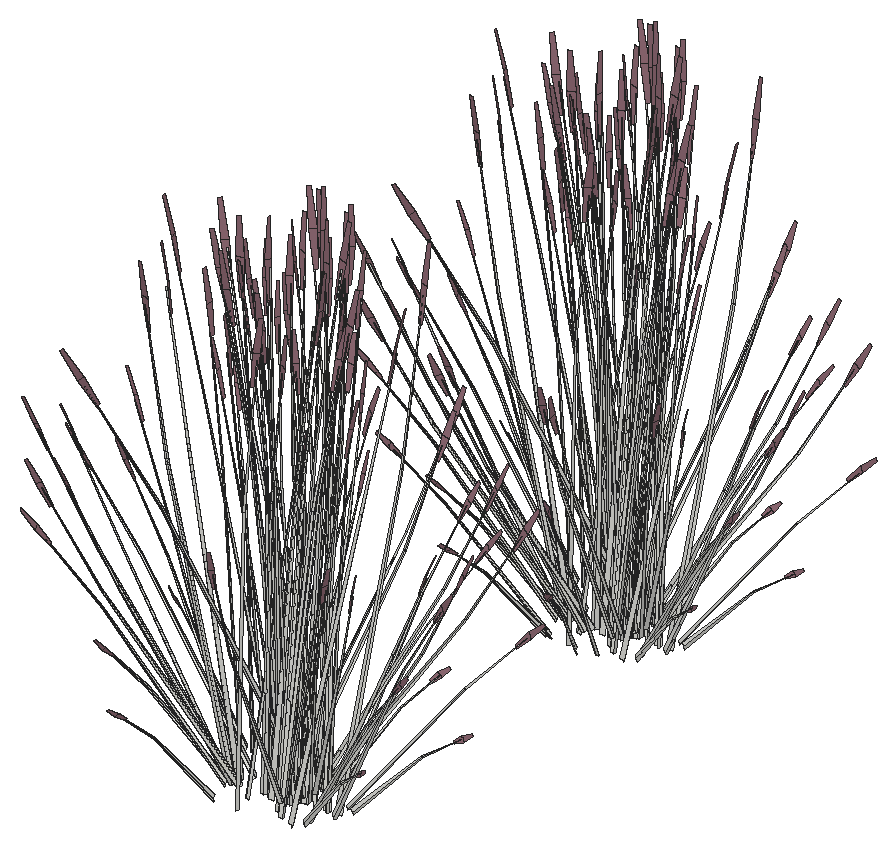
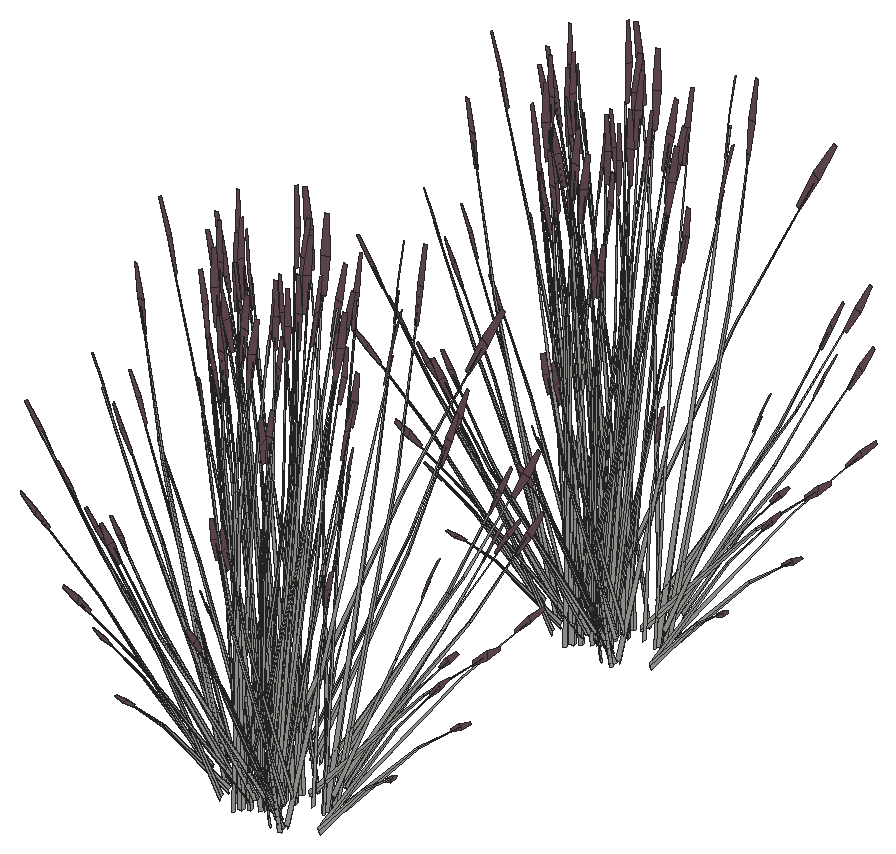
# SketchUp Ruby script. Lengths in inches.
U = 1.inch
M = Sketchup.active_model
def pt(a) = Geom::Point3d.new(a.map { |v| v * U })
def face(e, loops, mat)
  f = e.add_face(loops[0].map { |a| pt(a) })
  loops[1..].each { |l| e.add_face(l.map { |a| pt(a) }).erase! }
  f.material = f.back_material = mat if mat
  f
end
# faces: each face lists its corners as indices into pts; further lists are holes
def faces(e, pts, list, mat = nil) = list.each { |f| face(e, (f[0].is_a?(Array) ? f : [f]).map { |l| l.map { |i| pts[i] } }, mat) }
# xy, xz, yz: faces in a plane at the given z, y or x. An outline is a flat list of corners, or four numbers for a rectangle; further outlines are holes
def ring(l) = l.size == 4 ? [[l[0], l[1]], [l[2], l[1]], [l[2], l[3]], [l[0], l[3]]] : l.each_slice(2).to_a
def flat(e, list, mat, &to3) = list.each { |f| face(e, (f[0].is_a?(Array) ? f : [f]).map { |l| ring(l).map { |u, v| to3.(u, v) } }, mat) }
def xy(e, z, list, mat = nil) = flat(e, list, mat) { |x, y| [x, y, z] }
def xz(e, y, list, mat = nil) = flat(e, list, mat) { |x, z| [x, y, z] }
def yz(e, x, list, mat = nil) = flat(e, list, mat) { |y, z| [x, y, z] }
def lines(e, pts, list) = list.each { |a, b| e.add_line(pt(pts[a]), pt(pts[b])) }
# prism: a flat outline (further loops are holes) pulled along v
def prism(e, loops, v, mat = nil)
  f = face(e, loops, mat); d = Geom::Vector3d.new(v.map { |x| x * U })
  f.pushpull(f.normal.samedirection?(d) ? d.length : -d.length)
end
def box(e, o, s, mat = nil) = prism(e, [[o, [o[0] + s[0], o[1], o[2]], [o[0] + s[0], o[1] + s[1], o[2]], [o[0], o[1] + s[1], o[2]]]], [0, 0, s[2]], mat)
def at(x, y, z, deg = 0) = Geom::Transformation.translation(pt([x, y, z])) * Geom::Transformation.rotation(ORIGIN, Z_AXIS, deg.degrees)
def axes(o, x, y, z) = Geom::Transformation.new([*x, 0, *y, 0, *z, 0, *pt(o).to_a, 1])
def part(name) = M.definitions.add(name)
# library, detail: a bought-in or finely detailed component or shape, given as its bounding box
def library(name, o, s) = part(name).tap { |d| box(d.entities, o, s) }
def detail(e, o, s) = box(e.add_group.entities, o, s)
def put(e, d, t, mat = nil) = e.add_instance(d, t).tap { |i| i.material = mat if mat }
def group(e, t, mat = nil) = e.add_group.tap { |g| g.transformation = t; g.material = mat if mat }.entities
root = M.entities
M.materials.add("LightPink_Translucent").color = [144, 107, 117]
c1 = part("blade")
p = [[2.15,0.21,22],[0,0.17,0],[0.09,0.45,0],[2.18,0.31,22],[2.29,0.31,22],[0.38,0.45,0],
  [2.48,0.24,33],[2.49,0.24,33],[2.48,0.22,33]]
faces(c1.entities,p,[[0,1,2,3],[4,5,2,3],[6,3,4,7],[8,0,3,6]])
c2 = part("seeds")
p = [[0.3,-0.1,1.38],[-0.01,-0.03,1.59],[-0.01,-0.03,0.03],[0.14,-0.07,-0.07],[0.29,-0.03,3],[0.15,0.01,3.11]]
faces(c2.entities,p,[[0,1,2,3],[1,0,4,5]],"LightPink_Translucent")
c3 = part("blade with seeds")
put(c3.entities,c1,at(0,0,0))
put(c3.entities,c2,axes([2.4,0.25,30.99],[1.5799,-0.05474,1.17369],[-0.12525,1.92788,0.29478],[-0.07173,-0.02425,1.56792]))
put(root,c3,axes([55.18,640.24,46.68],[-0.87728,-0.69587,-0.51099],[0.92674,-0.60943,-0.3958],[0.13348,-0.35356,0.97773]))
put(root,c3,axes([48.84,638.0625,44.77],[0.63926,0.36046,1.1486],[-0.93099,0.21668,0.84392],[-0.1992,-0.27702,0.25299]))
put(root,c3,axes([50.39,639.97,46.98],[-1.04497,-0.50058,-0.71045],[0.74264,-0.8772,0.08574],[-0.3786,-0.29889,1.00501]))
put(root,c3,axes([49.9,640,46.68],[-1.20928,0.24619,-0.51099],[-0.21154,-0.93233,-0.3958],[-0.32481,-0.26718,0.97773]))
put(root,c3,axes([57.04,642.22,46.98],[0.64013,-0.81717,-0.71045],[1.12174,0.58074,0.08574],[0.38221,-0.29607,1.00501]))
put(root,c3,axes([50.12,639.84,44.375],[-0.7662,-1.03778,0],[1.28187,-0.57875,-0.51607],[0.29196,-0.13181,1.63711]))
put(root,c3,axes([57.01,641.84,46.68],[-0.31482,-0.94565,-0.51099],[1.19224,-0.16542,-0.3958],[0.34166,-0.254,0.97773]))
put(root,c3,axes([52.89,645.64,45.33],[1.05902,0.41762,1.51261],[-1.03748,0.89969,0.59816],[-0.46471,-0.53324,1.26806]))
put(root,c3,axes([57.97,641.47,44.59],[-0.4378,-0.03068,1.43002],[-0.44851,-0.8229,-0.30754],[0.53783,-0.23279,0.61141]))
put(root,c3,axes([58.47,639.96,44.77],[-0.40819,0.5272,1.1486],[-0.35086,-0.70831,0.84392],[0.33713,-0.17749,0.25299]))
put(root,c3,axes([47.01,643.53,44.375],[-1.53239,0,0],[0,-1.1575,-0.51607],[0,-0.26363,1.63711]))
put(root,c3,axes([47.27,641.47,44.59],[0.23927,0.28834,1.43002],[-0.55135,0.78376,-0.30754],[-0.56612,-0.18733,0.61141]))
put(root,c3,axes([48.26,641.21,46.98],[-1.22504,-0.02494,-0.71045],[0.08228,-1.05005,0.08574],[-0.51899,-0.11081,1.00501]))
put(root,c3,axes([48.19,643.23,44.33],[-1.1399,0.87071,0.30756],[-1.1406,-0.86155,-0.36492],[-0.03981,-0.24727,1.64885]))
put(root,c3,axes([51.82,643.63,44.43],[1.3808,0.50196,0.24065],[-0.66454,1.04299,0.50002],[0,-0.24043,1.60543]))
put(root,c3,axes([47.85,641.42,46.68],[-0.88986,0.68603,-0.51099],[-0.77932,-0.72471,-0.3958],[-0.45212,-0.10438,0.97773]))
put(root,c3,axes([45.84,642.33,44.77],[0.78239,-0.07411,1.1486],[-0.49629,0.65296,0.84392],[-0.38663,-0.09795,0.25299]))
put(root,c3,axes([51.375,642.94,44.72],[-1.33077,0.06393,0.44739],[-0.12035,-1.06125,-0.21531],[0.23824,-0.10756,1.43643]))
put(root,c3,axes([47.9375,643.71,44.48],[0,1.03566,0.49651],[-1.37109,0,0],[0,-0.23588,1.57504]))
put(root,c3,axes([57.5625,643.94,46.68],[0.332,-0.94205,-0.51099],[1.13828,0.3229,-0.3958],[0.45829,-0.08638,0.97773]))
put(root,c3,axes([55.76,640.1,44.375],[0.7662,-1.03778,0],[1.28187,0.57875,-0.51607],[0.29196,0.13181,1.63711]))
put(root,c3,axes([51.33,643.32,44.36],[0.53281,1.15808,0.45755],[-1.52239,0.4027,0.17955],[0.01861,-0.2128,1.58856]))
put(root,c3,axes([58.78,644.21,43.98],[-0.7893,0.12429,1.41583],[-0.12563,-0.9893,0.08104],[0.55282,-0.14974,0.80566]))
put(root,c3,axes([51.06,644.23,44.72],[-0.59459,0.93321,0.44739],[-1.23546,-0.44912,-0.21531],[0,-0.21512,1.43643]))
put(root,c3,axes([53.24,643.42,44.21],[0,-1.19833,0],[1.53239,0,0],[0,0,1.79456]))
put(root,c3,axes([55.1,640.65,44.48],[-1.14694,-0.51783,0.49651],[0.68554,-0.92854,0],[0.26122,0.11794,1.57504]))
put(root,c3,axes([57.34,644.28,46.98],[1.07686,-0.45739,-0.71045],[0.60013,0.94154,0.08574],[0.52031,-0.10696,1.00501]))
put(root,c3,axes([52.52,642.66,44.36],[-1.01611,0.93987,0.45755],[-1.20717,-0.82966,0.17955],[0.24496,-0.0938,1.58856]))
put(root,c3,axes([53.625,644.34,44.3],[-1.1399,-0.8914,-0.06131],[1.1406,-0.89194,0],[-0.03981,-0.03113,1.75571]))
put(root,c3,axes([50.75,641.11,44.47],[-0.35402,1.02926,0.17642],[-1.29548,-0.29127,0.35086],[0.22379,-0.00501,1.60407]))
put(root,c3,axes([53.46,642.26,44.62],[0.23642,-0.92427,0.1448],[1.15506,0.16044,-0.41347],[0.21021,0.09491,1.26744]))
put(root,c3,axes([51.46,644.45,44.36],[1.54892,0.2182,0.45755],[-0.31522,1.23236,0.17955],[-0.22636,-0.119,1.58856]))
put(root,c3,axes([52.96,642.5,44.72],[-0.73619,-0.86927,0.44739],[1.11511,-0.61213,-0.21531],[0.23824,0.10756,1.43643]))
put(root,c3,axes([50.63,646.42,44.47],[1.31687,-0.27488,0.17642],[0.32517,1.02297,0.35086],[-0.11745,-0.14905,1.60407]))
put(root,c3,axes([54.28,643.68,44.21],[1.37109,0,0],[0,1.07219,0],[0,0,1.78407]))
put(root,c3,axes([54.67,641.17,44.47],[-1.31687,0.27488,0.17642],[-0.32517,-1.02297,0.35086],[0.11745,0.14905,1.60407]))
put(root,c3,axes([53.84,643.14,44.38],[-1.54892,-0.2182,0.49198],[0.31522,-1.23236,0.19306],[0.22636,0.119,1.70813]))
put(root,c3,axes([52.61,646.18,44.2],[-0.39985,-0.89288,0],[1.1418,-0.31268,0],[0,0,1.54371]))
put(root,c3,axes([51.84,645.33,44.62],[-0.23642,0.92427,0.1448],[-1.15506,-0.16044,-0.41347],[-0.21021,-0.09491,1.26744]))
put(root,c3,axes([54.55,646.48,44.47],[0.35402,-1.02926,0.17642],[1.29548,0.29127,0.35086],[-0.22379,0.00501,1.60407]))
put(root,c3,axes([54.25,644.14,44.21],[0.85545,0.66896,0],[-0.85545,0.66896,0],[0,0,1.69266]))
put(root,c3,axes([49.39,642.89,45.34],[0.34834,-0.14982,1.77064],[0.12012,1.04605,0.13857],[-0.75452,0.1388,0.63284]))
put(root,c3,axes([56.57,643.85,44.47],[-0.96285,-0.75439,0.17642],[0.97031,-0.7317,0.35086],[-0.10634,0.15406,1.60407]))
put(root,c3,axes([60.42,644.54,44.77],[-0.75718,0.17097,1.1486],[0.35641,-0.70661,0.84392],[0.40168,0.04835,0.25299]))
put(root,c3,axes([52.32,646.58,44.2],[-1.23546,-0.46496,0],[0.59459,-0.96613,0],[0,0,1.62707]))
put(root,c3,axes([50.2,646.94,44.48],[1.14694,0.51783,0.49651],[-0.68554,0.92854,0],[-0.26122,-0.11794,1.57504]))
put(root,c3,axes([54.24,643.36,44.72],[0.59459,-0.93321,0.44739],[1.23546,0.44912,-0.21531],[0,0.21512,1.43643]))
put(root,c3,axes([54.01,643.89,44.29],[0,1.19774,-0.05637],[-1.53239,0,0],[0,0.03764,1.79368]))
put(root,c3,axes([46.99,643.46,46.68],[-0.332,0.94205,-0.51099],[-1.13828,-0.3229,-0.3958],[-0.45829,0.08638,0.97773]))
put(root,c3,axes([49.54,647.49,44.375],[-0.7662,1.03778,0],[-1.28187,-0.57875,-0.51607],[-0.29196,-0.13181,1.63711]))
put(root,c3,axes([57.36,643.88,44.48],[0,-1.03566,0.49651],[1.37109,0,0],[0,0.23588,1.57504]))
put(root,c3,axes([53.93,644.66,44.72],[1.33077,-0.06393,0.44739],[0.12035,1.06125,-0.21531],[-0.23824,0.10756,1.43643]))
put(root,c3,axes([54.76,643.57,44.62],[1.1418,-0.30203,0.1448],[0.39985,0.86246,-0.41347],[0,0.18981,1.26744]))
put(root,c3,axes([59,645.68,44.59],[-0.29514,-0.25472,1.43002],[0.38401,-0.84262,-0.30754],[0.59714,0.11414,0.61141]))
put(root,c3,axes([53.72,646.6,44.2],[1.23546,0.46496,0],[-0.59459,0.96613,0],[0,0,1.74954]))
put(root,c3,axes([54.22,647.63,44.19],[-0.75665,-1.04141,-0.05142],[1.28187,-0.57875,0.51607],[-0.31588,0.09915,1.6363]))
put(root,c3,axes([53.95,645.11,44.62],[0.90538,0.62224,0.1448],[-0.75521,0.70202,-0.41347],[-0.21021,0.09491,1.26744]))
put(root,c3,axes([56.29,646.1875,46.98],[1.22504,0.02494,-0.71045],[-0.08228,1.05005,0.08574],[0.51899,0.11081,1.00501]))
put(root,c3,axes([54.91,647.03,44.48],[1.14694,-0.51783,0.49651],[0.68554,0.92854,0],[-0.26122,0.11794,1.57504]))
put(root,c3,axes([53.28,646.21,44.29],[0.53281,1.18979,-0.06012],[-1.52239,0.41691,0],[0.01861,0.04155,1.72173]))
put(root,c3,axes([45.62,645.67,44.59],[0.42589,0.08502,1.43002],[0.2745,0.86839,-0.30754],[-0.57851,0.16255,0.61141]))
put(root,c3,axes([58.29,644.06,44.375],[1.53239,0,0],[0,1.1575,-0.51607],[0,0.26363,1.63711]))
put(root,c3,axes([57.68,644.65,44.2],[-1.53164,-0.00828,-0.04976],[0,-1.1575,0.49943],[-0.04813,0.2635,1.58352]))
put(root,c3,axes([44.73,647.49,44.77],[0.51072,-0.46938,1.1486],[0.20153,0.74307,0.84392],[-0.36908,0.13305,0.25299]))
put(root,c3,axes([54.25,647.1,44.33],[1.53422,0.33662,0.30756],[-0.38383,1.20322,-0.36492],[-0.25393,0.15059,1.64885]))
put(root,c3,axes([56.21,646.99,44.77],[-0.69001,-0.29779,1.1486],[0.89096,-0.30257,0.84392],[0.24031,0.2563,0.25299]))
put(root,c3,axes([47.54,645.56,46.68],[0.31482,0.94565,-0.51099],[-1.19224,0.16542,-0.3958],[-0.34166,0.254,0.97773]))
put(root,c3,axes([55.18,647.75,44.375],[0.7662,1.03778,0],[-1.28187,0.57875,-0.51607],[-0.29196,0.13181,1.63711]))
put(root,c3,axes([54.53,643.64,44.84],[-0.03348,-0.97511,1.41272],[1.51511,0.25277,0.59816],[-0.35835,0.53357,1.3335]))
put(root,c3,axes([54.65,647.4,46.68],[1.20928,-0.24619,-0.51099],[0.21154,0.93233,-0.3958],[0.32481,0.26718,0.97773]))
put(root,c3,axes([56.32,648.35,44.67],[-0.78586,-0.03248,1.0506],[0.51898,-0.68985,0.58006],[0.31045,0.24509,0.8241]))
put(root,c3,axes([53.75,646.67,44.59],[0.02163,-0.34331,1.43002],[1.03345,-0.38348,-0.30754],[0.31903,0.4109,0.61141]))
put(root,c3,axes([49.07,649.53,44.77],[-0.03171,-0.6158,1.1486],[0.7925,0.43922,0.84392],[-0.15586,0.29352,0.25299]))
put(root,c3,axes([49.36,647.16,47],[0.87728,0.69587,-0.5672],[-0.92674,0.60943,-0.43934],[-0.13348,0.35356,1.08528]))
put(root,c3,axes([48.41,648.2,44.82],[1.11329,-0.1834,0.06507],[0.25594,0.73887,-0.86304],[-0.07058,0.37403,0.7736]))
put(root,c3,axes([51.96,647.83,46.68],[1.20468,0.25962,-0.51099],[-0.41292,0.89013,-0.3958],[0.11046,0.35838,0.97773]))
put(root,c3,axes([49.09,646.84,47.34],[-0.03189,0.95798,-0.7886],[-1.34277,-0.06434,0.09517],[-0.14171,0.40585,1.11556]))
put(root,c3,axes([51.53,647.66,46.98],[0.5849,0.8421,-0.71045],[-1.20401,0.4693,0.08574],[0.13677,0.40688,1.00501]))
put(root,c3,axes([48.14,648.99,44.59],[0.38672,-0.16338,1.43002],[0.95481,0.49262,-0.30754],[-0.28419,0.42626,0.61141]))
put(root,c3,axes([48.64,648.19,45.36],[0.02693,-0.53464,1.54345],[1.21102,0.2824,0.21329],[-0.10493,0.5698,0.72882]))
put(root,c3,axes([59.15,683.33,44.59],[-0.34835,0.20963,1.43002],[-1.04325,-0.36691,-0.30754],[0.19338,-0.4563,0.61141]))
put(root,c3,axes([57.5625,684.0625,46.98],[-0.5849,-0.8421,-0.71045],[1.20401,-0.4693,0.08574],[-0.13677,-0.40688,1.00501]))
put(root,c3,axes([53.76,682.9375,44.59],[-0.07421,0.33879,1.43002],[-1.08488,0.28361,-0.30754],[-0.25359,-0.4379,0.61141]))
put(root,c3,axes([60,684.89,46.98],[0.03189,-0.95798,-0.71045],[1.34277,0.06434,0.08574],[0.14171,-0.40585,1.00501]))
put(root,c3,axes([57.12,683.89,46.68],[-1.20468,-0.25962,-0.51099],[0.41292,-0.89013,-0.3958],[-0.11046,-0.35838,0.97773]))
put(root,c3,axes([57.87,681.66,44.77],[0.15721,0.60392,1.1486],[-0.87211,-0.33448,0.84392],[0.09385,-0.30923,0.25299]))
put(root,c3,axes([59.72,684.57,46.68],[-0.87728,-0.69587,-0.51099],[0.92674,-0.60943,-0.3958],[0.13348,-0.35356,0.97773]))
put(root,c3,axes([53.38,682.39,44.77],[0.63926,0.36046,1.1486],[-0.93099,0.21668,0.84392],[-0.1992,-0.27702,0.25299]))
put(root,c3,axes([54.93,684.3,46.98],[-1.04497,-0.50058,-0.71045],[0.74264,-0.8772,0.08574],[-0.3786,-0.29889,1.00501]))
put(root,c3,axes([54.4375,684.33,46.68],[-1.20928,0.24619,-0.51099],[-0.21154,-0.93233,-0.3958],[-0.32481,-0.26718,0.97773]))
put(root,c3,axes([61.58,686.55,46.98],[0.64013,-0.81717,-0.71045],[1.12174,0.58074,0.08574],[0.38221,-0.29607,1.00501]))
put(root,c3,axes([54.66,684.17,44.375],[-0.7662,-1.03778,0],[1.28187,-0.57875,-0.51607],[0.29196,-0.13181,1.63711]))
put(root,c3,axes([61.55,686.17,46.68],[-0.31482,-0.94565,-0.51099],[1.19224,-0.16542,-0.3958],[0.34166,-0.254,0.97773]))
put(root,c3,axes([57.43,689.96,45.33],[1.05902,0.41762,1.51261],[-1.03748,0.89969,0.59816],[-0.46471,-0.53324,1.26806]))
put(root,c3,axes([62.51,685.8,44.59],[-0.4378,-0.03068,1.43002],[-0.44851,-0.8229,-0.30754],[0.53783,-0.23279,0.61141]))
put(root,c3,axes([63.01,684.29,44.77],[-0.40819,0.5272,1.1486],[-0.35086,-0.70831,0.84392],[0.33713,-0.17749,0.25299]))
put(root,c3,axes([51.55,687.86,44.375],[-1.53239,0,0],[0,-1.1575,-0.51607],[0,-0.26363,1.63711]))
put(root,c3,axes([51.81,685.79,44.59],[0.23927,0.28834,1.43002],[-0.55135,0.78376,-0.30754],[-0.56612,-0.18733,0.61141]))
put(root,c3,axes([52.8,685.54,46.98],[-1.22504,-0.02494,-0.71045],[0.08228,-1.05005,0.08574],[-0.51899,-0.11081,1.00501]))
put(root,c3,axes([52.73,687.56,44.33],[-1.1399,0.87071,0.30756],[-1.1406,-0.86155,-0.36492],[-0.03981,-0.24727,1.64885]))
put(root,c3,axes([56.36,687.96,44.43],[1.3808,0.50196,0.24065],[-0.66454,1.04299,0.50002],[0,-0.24043,1.60543]))
put(root,c3,axes([52.39,685.75,46.68],[-0.88986,0.68603,-0.51099],[-0.77932,-0.72471,-0.3958],[-0.45212,-0.10438,0.97773]))
put(root,c3,axes([50.38,686.66,44.77],[0.78239,-0.07411,1.1486],[-0.49629,0.65296,0.84392],[-0.38663,-0.09795,0.25299]))
put(root,c3,axes([55.91,687.26,44.72],[-1.33077,0.06393,0.44739],[-0.12035,-1.06125,-0.21531],[0.23824,-0.10756,1.43643]))
put(root,c3,axes([52.48,688.04,44.48],[0,1.03566,0.49651],[-1.37109,0,0],[0,-0.23588,1.57504]))
put(root,c3,axes([62.1,688.27,46.68],[0.332,-0.94205,-0.51099],[1.13828,0.3229,-0.3958],[0.45829,-0.08638,0.97773]))
put(root,c3,axes([60.3,684.43,44.375],[0.7662,-1.03778,0],[1.28187,0.57875,-0.51607],[0.29196,0.13181,1.63711]))
put(root,c3,axes([55.87,687.65,44.36],[0.53281,1.15808,0.45755],[-1.52239,0.4027,0.17955],[0.01861,-0.2128,1.58856]))
put(root,c3,axes([63.32,688.53,43.98],[-0.7893,0.12429,1.41583],[-0.12563,-0.9893,0.08104],[0.55282,-0.14974,0.80566]))
put(root,c3,axes([55.6,688.56,44.72],[-0.59459,0.93321,0.44739],[-1.23546,-0.44912,-0.21531],[0,-0.21512,1.43643]))
put(root,c3,axes([57.78,687.74,44.21],[0,-1.19833,0],[1.53239,0,0],[0,0,1.79456]))
put(root,c3,axes([59.64,684.98,44.48],[-1.14694,-0.51783,0.49651],[0.68554,-0.92854,0],[0.26122,0.11794,1.57504]))
put(root,c3,axes([61.88,688.61,46.98],[1.07686,-0.45739,-0.71045],[0.60013,0.94154,0.08574],[0.52031,-0.10696,1.00501]))
put(root,c3,axes([57.06,686.99,44.36],[-1.01611,0.93987,0.45755],[-1.20717,-0.82966,0.17955],[0.24496,-0.0938,1.58856]))
put(root,c3,axes([58.17,688.67,44.3],[-1.1399,-0.8914,-0.06131],[1.1406,-0.89194,0],[-0.03981,-0.03113,1.75571]))
put(root,c3,axes([55.29,685.44,44.47],[-0.35402,1.02926,0.17642],[-1.29548,-0.29127,0.35086],[0.22379,-0.00501,1.60407]))
put(root,c3,axes([58,686.59,44.62],[0.23642,-0.92427,0.1448],[1.15506,0.16044,-0.41347],[0.21021,0.09491,1.26744]))
put(root,c3,axes([56,688.78,44.36],[1.54892,0.2182,0.45755],[-0.31522,1.23236,0.17955],[-0.22636,-0.119,1.58856]))
put(root,c3,axes([57.5,686.83,44.72],[-0.73619,-0.86927,0.44739],[1.11511,-0.61213,-0.21531],[0.23824,0.10756,1.43643]))
put(root,c3,axes([55.17,690.75,44.47],[1.31687,-0.27488,0.17642],[0.32517,1.02297,0.35086],[-0.11745,-0.14905,1.60407]))
put(root,c3,axes([58.82,688.01,44.21],[1.37109,0,0],[0,1.07219,0],[0,0,1.78407]))
put(root,c3,axes([59.21,685.5,44.47],[-1.31687,0.27488,0.17642],[-0.32517,-1.02297,0.35086],[0.11745,0.14905,1.60407]))
put(root,c3,axes([58.38,687.47,44.38],[-1.54892,-0.2182,0.49198],[0.31522,-1.23236,0.19306],[0.22636,0.119,1.70813]))
put(root,c3,axes([57.15,690.51,44.2],[-0.39985,-0.89288,0],[1.1418,-0.31268,0],[0,0,1.54371]))
put(root,c3,axes([56.38,689.66,44.62],[-0.23642,0.92427,0.1448],[-1.15506,-0.16044,-0.41347],[-0.21021,-0.09491,1.26744]))
put(root,c3,axes([59.09,690.81,44.47],[0.35402,-1.02926,0.17642],[1.29548,0.29127,0.35086],[-0.22379,0.00501,1.60407]))
put(root,c3,axes([58.79,688.47,44.21],[0.85545,0.66896,0],[-0.85545,0.66896,0],[0,0,1.69266]))
put(root,c3,axes([53.93,687.22,45.34],[0.34834,-0.14982,1.77064],[0.12012,1.04605,0.13857],[-0.75452,0.1388,0.63284]))
put(root,c3,axes([61.11,688.18,44.47],[-0.96285,-0.75439,0.17642],[0.97031,-0.7317,0.35086],[-0.10634,0.15406,1.60407]))
put(root,c3,axes([64.96,688.87,44.77],[-0.75718,0.17097,1.1486],[0.35641,-0.70661,0.84392],[0.40168,0.04835,0.25299]))
put(root,c3,axes([56.86,690.91,44.2],[-1.23546,-0.46496,0],[0.59459,-0.96613,0],[0,0,1.62707]))
put(root,c3,axes([54.74,691.27,44.48],[1.14694,0.51783,0.49651],[-0.68554,0.92854,0],[-0.26122,-0.11794,1.57504]))
put(root,c3,axes([58.78,687.6875,44.72],[0.59459,-0.93321,0.44739],[1.23546,0.44912,-0.21531],[0,0.21512,1.43643]))
put(root,c3,axes([58.55,688.22,44.29],[0,1.19774,-0.05637],[-1.53239,0,0],[0,0.03764,1.79368]))
put(root,c3,axes([51.53,687.79,46.68],[-0.332,0.94205,-0.51099],[-1.13828,-0.3229,-0.3958],[-0.45829,0.08638,0.97773]))
put(root,c3,axes([54.08,691.81,44.375],[-0.7662,1.03778,0],[-1.28187,-0.57875,-0.51607],[-0.29196,-0.13181,1.63711]))
put(root,c3,axes([61.9,688.21,44.48],[0,-1.03566,0.49651],[1.37109,0,0],[0,0.23588,1.57504]))
put(root,c3,axes([58.47,688.98,44.72],[1.33077,-0.06393,0.44739],[0.12035,1.06125,-0.21531],[-0.23824,0.10756,1.43643]))
put(root,c3,axes([59.3,687.9,44.62],[1.1418,-0.30203,0.1448],[0.39985,0.86246,-0.41347],[0,0.18981,1.26744]))
put(root,c3,axes([63.54,690,44.59],[-0.29514,-0.25472,1.43002],[0.38401,-0.84262,-0.30754],[0.59714,0.11414,0.61141]))
put(root,c3,axes([58.26,690.93,44.2],[1.23546,0.46496,0],[-0.59459,0.96613,0],[0,0,1.74954]))
put(root,c3,axes([58.76,691.96,44.19],[-0.75665,-1.04141,-0.05142],[1.28187,-0.57875,0.51607],[-0.31588,0.09915,1.6363]))
put(root,c3,axes([58.49,689.44,44.62],[0.90538,0.62224,0.1448],[-0.75521,0.70202,-0.41347],[-0.21021,0.09491,1.26744]))
put(root,c3,axes([60.83,690.52,46.98],[1.22504,0.02494,-0.71045],[-0.08228,1.05005,0.08574],[0.51899,0.11081,1.00501]))
put(root,c3,axes([59.45,691.36,44.48],[1.14694,-0.51783,0.49651],[0.68554,0.92854,0],[-0.26122,0.11794,1.57504]))
put(root,c3,axes([57.82,690.54,44.29],[0.53281,1.18979,-0.06012],[-1.52239,0.41691,0],[0.01861,0.04155,1.72173]))
put(root,c3,axes([50.16,690,44.59],[0.42589,0.08502,1.43002],[0.2745,0.86839,-0.30754],[-0.57851,0.16255,0.61141]))
put(root,c3,axes([62.83,688.39,44.375],[1.53239,0,0],[0,1.1575,-0.51607],[0,0.26363,1.63711]))
put(root,c3,axes([62.22,688.98,44.2],[-1.53164,-0.00828,-0.04976],[0,-1.1575,0.49943],[-0.04813,0.2635,1.58352]))
put(root,c3,axes([49.27,691.82,44.77],[0.51072,-0.46938,1.1486],[0.20153,0.74307,0.84392],[-0.36908,0.13305,0.25299]))
put(root,c3,axes([58.79,691.42,44.33],[1.53422,0.33662,0.30756],[-0.38383,1.20322,-0.36492],[-0.25393,0.15059,1.64885]))
put(root,c3,axes([60.75,691.32,44.77],[-0.69001,-0.29779,1.1486],[0.89096,-0.30257,0.84392],[0.24031,0.2563,0.25299]))
put(root,c3,axes([52.08,689.89,46.68],[0.31482,0.94565,-0.51099],[-1.19224,0.16542,-0.3958],[-0.34166,0.254,0.97773]))
put(root,c3,axes([59.72,692.08,44.375],[0.7662,1.03778,0],[-1.28187,0.57875,-0.51607],[-0.29196,0.13181,1.63711]))
put(root,c3,axes([59.07,687.97,44.84],[-0.03348,-0.97511,1.41272],[1.51511,0.25277,0.59816],[-0.35835,0.53357,1.3335]))
put(root,c3,axes([59.19,691.73,46.68],[1.20928,-0.24619,-0.51099],[0.21154,0.93233,-0.3958],[0.32481,0.26718,0.97773]))
put(root,c3,axes([60.86,692.67,44.67],[-0.78586,-0.03248,1.0506],[0.51898,-0.68985,0.58006],[0.31045,0.24509,0.8241]))
put(root,c3,axes([58.29,691,44.59],[0.02163,-0.34331,1.43002],[1.03345,-0.38348,-0.30754],[0.31903,0.4109,0.61141]))
put(root,c3,axes([53.61,693.86,44.77],[-0.03171,-0.6158,1.1486],[0.7925,0.43922,0.84392],[-0.15586,0.29352,0.25299]))
put(root,c3,axes([53.9,691.49,47],[0.87728,0.69587,-0.5672],[-0.92674,0.60943,-0.43934],[-0.13348,0.35356,1.08528]))
put(root,c3,axes([52.95,692.53,44.82],[1.11329,-0.1834,0.06507],[0.25594,0.73887,-0.86304],[-0.07058,0.37403,0.7736]))
put(root,c3,axes([56.5,692.16,46.68],[1.20468,0.25962,-0.51099],[-0.41292,0.89013,-0.3958],[0.11046,0.35838,0.97773]))
put(root,c3,axes([53.63,691.17,47.34],[-0.03189,0.95798,-0.7886],[-1.34277,-0.06434,0.09517],[-0.14171,0.40585,1.11556]))
put(root,c3,axes([56.07,691.99,46.98],[0.5849,0.8421,-0.71045],[-1.20401,0.4693,0.08574],[0.13677,0.40688,1.00501]))
put(root,c3,axes([52.68,693.32,44.59],[0.38672,-0.16338,1.43002],[0.95481,0.49262,-0.30754],[-0.28419,0.42626,0.61141]))
put(root,c3,axes([53.18,692.52,45.36],[0.02693,-0.53464,1.54345],[1.21102,0.2824,0.21329],[-0.10493,0.5698,0.72882]))
